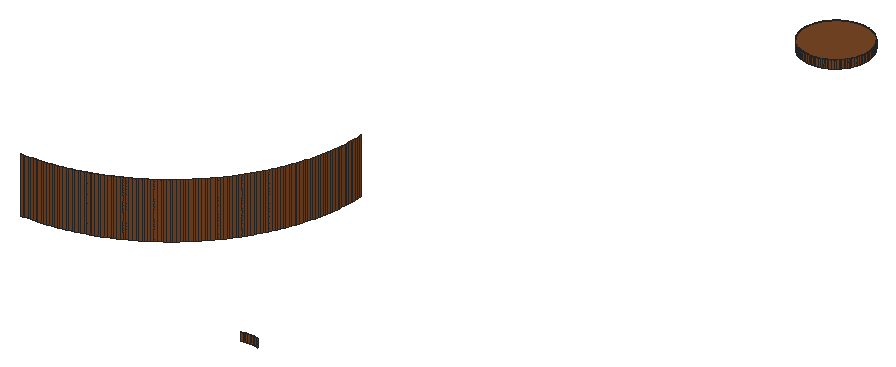
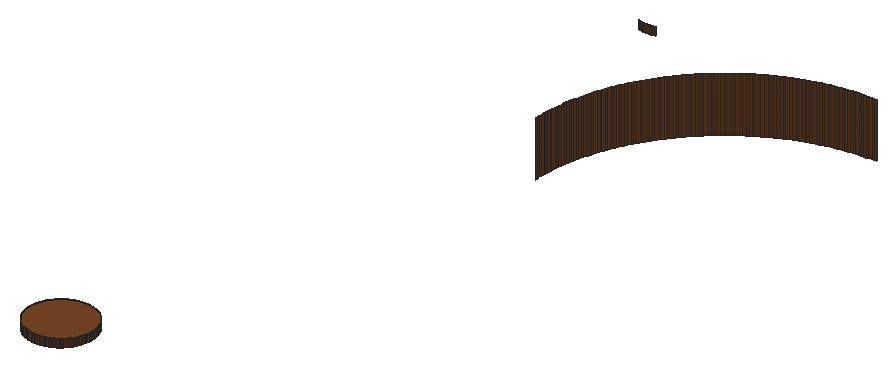
# SketchUp Ruby script. Lengths in inches.
U = 1.inch
M = Sketchup.active_model
def pt(a) = Geom::Point3d.new(a.map { |v| v * U })
def face(e, loops, mat)
  f = e.add_face(loops[0].map { |a| pt(a) })
  loops[1..].each { |l| e.add_face(l.map { |a| pt(a) }).erase! }
  f.material = f.back_material = mat if mat
  f
end
# faces: each face lists its corners as indices into pts; further lists are holes
def faces(e, pts, list, mat = nil) = list.each { |f| face(e, (f[0].is_a?(Array) ? f : [f]).map { |l| l.map { |i| pts[i] } }, mat) }
# xy, xz, yz: faces in a plane at the given z, y or x. An outline is a flat list of corners, or four numbers for a rectangle; further outlines are holes
def ring(l) = l.size == 4 ? [[l[0], l[1]], [l[2], l[1]], [l[2], l[3]], [l[0], l[3]]] : l.each_slice(2).to_a
def flat(e, list, mat, &to3) = list.each { |f| face(e, (f[0].is_a?(Array) ? f : [f]).map { |l| ring(l).map { |u, v| to3.(u, v) } }, mat) }
def xy(e, z, list, mat = nil) = flat(e, list, mat) { |x, y| [x, y, z] }
def xz(e, y, list, mat = nil) = flat(e, list, mat) { |x, z| [x, y, z] }
def yz(e, x, list, mat = nil) = flat(e, list, mat) { |y, z| [x, y, z] }
def lines(e, pts, list) = list.each { |a, b| e.add_line(pt(pts[a]), pt(pts[b])) }
# prism: a flat outline (further loops are holes) pulled along v
def prism(e, loops, v, mat = nil)
  f = face(e, loops, mat); d = Geom::Vector3d.new(v.map { |x| x * U })
  f.pushpull(f.normal.samedirection?(d) ? d.length : -d.length)
end
def box(e, o, s, mat = nil) = prism(e, [[o, [o[0] + s[0], o[1], o[2]], [o[0] + s[0], o[1] + s[1], o[2]], [o[0], o[1] + s[1], o[2]]]], [0, 0, s[2]], mat)
def at(x, y, z, deg = 0) = Geom::Transformation.translation(pt([x, y, z])) * Geom::Transformation.rotation(ORIGIN, Z_AXIS, deg.degrees)
def axes(o, x, y, z) = Geom::Transformation.new([*x, 0, *y, 0, *z, 0, *pt(o).to_a, 1])
def part(name) = M.definitions.add(name)
# library, detail: a bought-in or finely detailed component or shape, given as its bounding box
def library(name, o, s) = part(name).tap { |d| box(d.entities, o, s) }
def detail(e, o, s) = box(e.add_group.entities, o, s)
def put(e, d, t, mat = nil) = e.add_instance(d, t).tap { |i| i.material = mat if mat }
def group(e, t, mat = nil) = e.add_group.tap { |g| g.transformation = t; g.material = mat if mat }.entities
root = M.entities
M.materials.add("[Wood Veneer 01]3").color = [120, 70, 37]
xy(root,118.5,[[146.99,81.33,146.9,81.34,146.82,81.34,146.74,81.35,146.65,81.36,146.41,81.42,146.17,81.51,146.1,81.55,146.02,81.59,145.95,81.63,145.88,81.68,145.8125,81.72,145.75,81.77,145.68,81.83,145.62,81.89,145.5625,81.94,145.5,82.01,145.45,82.07,145.4,82.14,145.35,82.2,145.3,82.27,145.26,82.35,145.18,82.49,145.09,82.73,145.03,82.97,145.02,83.06,145,83.22,145,83.47,145.01,83.56,145.02,83.64,145.1,83.96,145.16,84.12,145.2,84.2,145.23,84.27,145.27,84.35,145.37,84.49,145.42,84.55,145.47,84.62,145.52,84.68,145.7,84.86,145.84,84.96,145.9,85.01,145.98,85.05,146.05,85.09,146.2,85.17,146.36,85.23,146.68,85.31,146.76,85.32,146.85,85.33,147.18,85.33,147.26,85.32,147.35,85.3,147.43,85.29,147.51,85.27,147.59,85.24,147.67,85.22,147.75,85.1875,147.83,85.15,147.9,85.12,147.98,85.08,148.05,85.04,148.12,84.99,148.1875,84.94,148.25,84.89,148.32,84.84,148.38,84.78,148.4375,84.72,148.5,84.66,148.55,84.6,148.7,84.39,148.78,84.25,148.82,84.17,148.85,84.1,148.88,84.02,148.91,83.9375,148.93,83.86,148.95,83.78,148.97,83.69,148.99,83.53,149,83.44,149,83.19,148.98,83.03,148.96,82.94,148.9,82.7,148.84,82.55,148.8,82.47,148.77,82.39,148.73,82.32,148.58,82.11,148.53,82.05,148.48,81.98,148.42,81.92,148.36,81.87,148.3,81.81,148.16,81.71,148.1,81.66,148.02,81.62,147.95,81.57,147.875,81.54,147.8,81.5,147.56,81.41,147.48,81.39,147.32,81.36,147.24,81.35,147.15,81.34,147.07,81.33]],"[Wood Veneer 01]3")
xz(root,41.99,[[142.76,118,142.85,118.5]],"[Wood Veneer 01]3")
xz(root,42,[[142.93,118,143.01,118.5],[143.01,118,143.1,118.5]],"[Wood Veneer 01]3")
xz(root,45,[[126,118,126.16,121.5],[126.16,118,126.3125,121.5]],"[Wood Veneer 01]3")
xz(root,81.33,[[146.99,118,147.07,118.5]],"[Wood Veneer 01]3")
xz(root,81.34,[[146.82,118,146.9,118.5]],"[Wood Veneer 01]3")
xz(root,85.33,[[146.85,118,146.93,118.5],[146.93,118,147.01,118.5],[147.01,118,147.1,118.5],[147.1,118,147.18,118.5]],"[Wood Veneer 01]3")
yz(root,138,[[56.6875,118,56.84,121.5],[56.84,118,57,121.5]],"[Wood Veneer 01]3")
yz(root,145,[[83.22,118,83.31,118.5],[83.31,118,83.39,118.5],[83.39,118,83.47,118.5]],"[Wood Veneer 01]3")
yz(root,149,[[83.19,118,83.28,118.5],[83.28,118,83.36,118.5],[83.36,118,83.44,118.5]],"[Wood Veneer 01]3")
p = [[142.44,41.92,118],[142.52,41.94,118],[142.52,41.94,118.5],[142.44,41.92,118.5],[142.6,41.96,118],[142.6,41.96,118.5],
  [143.43,41.95,118],[143.51,41.93,118],[143.51,41.93,118.5],[143.43,41.95,118.5],[142.68,41.97,118],[142.68,41.97,118.5],
  [142.76,41.99,118],[142.76,41.99,118.5],[142.85,41.99,118],[142.93,42,118],[142.93,42,118.5],[142.85,41.99,118.5],
  [143.1,42,118],[143.18,41.99,118],[143.18,41.99,118.5],[143.1,42,118.5],[143.26,41.98,118],[143.26,41.98,118.5],
  [143.35,41.97,118],[143.35,41.97,118.5],[126.3125,45,118],[126.3125,45,121],[126.3125,45,121.5],[126.47,45.01,121.5],
  [126.47,45.01,121],[126.47,45.01,118],[126.63,45.02,121.5],[126.63,45.02,121],[126.63,45.02,118],[126.78,45.03,121.5],
  [126.78,45.03,121],[126.78,45.03,118],[126.94,45.04,121.5],[126.94,45.04,121],[126.94,45.04,118],[127.1,45.05,121.5],
  [127.1,45.05,121],[127.1,45.05,118],[127.25,45.07,121.5],[127.25,45.07,121],[127.25,45.07,118],[127.41,45.08,121.5],
  [127.41,45.08,121],[127.41,45.08,118],[127.57,45.1,121.5],[127.57,45.1,121],[127.57,45.1,118],[127.72,45.125,121.5],
  [127.72,45.125,121],[127.72,45.125,118],[127.88,45.15,121.5],[127.88,45.15,121],[127.88,45.15,118],[128.03,45.17,121.5],
  [128.03,45.17,121],[128.03,45.17,118],[128.1875,45.2,121.5],[128.1875,45.2,121],[128.1875,45.2,118],[128.34,45.23,121.5],
  [128.34,45.23,121],[128.34,45.23,118],[128.49,45.26,121.5],[128.49,45.26,121],[128.49,45.26,118],[128.65,45.3,121.5],
  [128.65,45.3,121],[128.65,45.3,118],[128.8,45.33,121.5],[128.8,45.33,121],[128.8,45.33,118],[128.95,45.37,121.5],
  [128.95,45.37,121],[128.95,45.37,118],[129.11,45.41,121.5],[129.11,45.41,121],[129.11,45.41,118],[129.26,45.45,121.5],
  [129.26,45.45,121],[129.26,45.45,118],[129.41,45.49,121.5],[129.41,45.49,121],[129.41,45.49,118],[129.56,45.54,121.5],
  [129.56,45.54,121],[129.56,45.54,118],[129.71,45.59,121.5],[129.71,45.59,121],[129.71,45.59,118],[129.86,45.64,121.5],
  [129.86,45.64,121],[129.86,45.64,118],[130.01,45.6875,121.5],[130.01,45.6875,121],[130.01,45.6875,118],[130.15,45.74,121.5],
  [130.15,45.74,121],[130.15,45.74,118],[130.3,45.8,121.5],[130.3,45.8,121],[130.3,45.8,118],[130.45,45.85,121.5],
  [130.45,45.85,121],[130.45,45.85,118],[130.59,45.91,121.5],[130.59,45.91,121],[130.59,45.91,118],[130.74,45.97,121.5],
  [130.74,45.97,121],[130.74,45.97,118],[130.88,46.04,121.5],[130.88,46.04,121],[130.88,46.04,118],[131.02,46.1,121.5],
  [131.02,46.1,121],[131.02,46.1,118],[131.17,46.17,121.5],[131.17,46.17,121],[131.17,46.17,118],[131.31,46.24,121.5],
  [131.31,46.24,121],[131.31,46.24,118],[131.45,46.31,121.5],[131.45,46.31,121],[131.45,46.31,118],[131.59,46.38,121.5],
  [131.59,46.38,121],[131.59,46.38,118],[131.73,46.45,121.5],[131.73,46.45,121],[131.73,46.45,118],[131.86,46.53,121.5],
  [131.86,46.53,121],[131.86,46.53,118],[132,46.61,121.5],[132,46.61,121],[132,46.61,118],[132.14,46.6875,121.5],
  [132.14,46.6875,121],[132.14,46.6875,118],[132.27,46.77,121.5],[132.27,46.77,121],[132.27,46.77,118],[132.4,46.85,121.5],
  [132.4,46.85,121],[132.4,46.85,118],[132.54,46.9375,121.5],[132.54,46.9375,121],[132.54,46.9375,118],[132.67,47.02,121.5],
  [132.67,47.02,121],[132.67,47.02,118],[132.8,47.11,121.5],[132.8,47.11,121],[132.8,47.11,118],[132.93,47.2,121.5],
  [132.93,47.2,121],[132.93,47.2,118],[133.05,47.29,121.5],[133.05,47.29,121],[133.05,47.29,118],[133.18,47.38,121.5],
  [133.18,47.38,121],[133.18,47.38,118],[133.31,47.48,121.5],[133.31,47.48,121],[133.31,47.48,118],[133.43,47.58,121.5],
  [133.43,47.58,121],[133.43,47.58,118],[133.55,47.67,121.5],[133.55,47.67,121],[133.55,47.67,118],[133.67,47.77,121.5],
  [133.67,47.77,121],[133.67,47.77,118],[133.79,47.875,121.5],[133.79,47.875,121],[133.79,47.875,118],[133.91,47.98,121.5],
  [133.91,47.98,121],[133.91,47.98,118],[134.03,48.08,121.5],[134.03,48.08,121],[134.03,48.08,118],[134.15,48.1875,121.5],
  [134.15,48.1875,121],[134.15,48.1875,118],[134.26,48.3,121.5],[134.26,48.3,121],[134.26,48.3,118],[134.375,48.4,121.5],
  [134.375,48.4,121],[134.375,48.4,118],[134.49,48.51,121.5],[134.49,48.51,121],[134.49,48.51,118],[134.6,48.625,121.5],
  [134.6,48.625,121],[134.6,48.625,118],[134.7,48.74,121.5],[134.7,48.74,121],[134.7,48.74,118],[134.8125,48.85,121.5],
  [134.8125,48.85,121],[134.8125,48.85,118],[134.92,48.97,121.5],[134.92,48.97,121],[134.92,48.97,118],[135.02,49.09,121.5],
  [135.02,49.09,121],[135.02,49.09,118],[135.125,49.21,121.5],[135.125,49.21,121],[135.125,49.21,118],[135.23,49.33,121.5],
  [135.23,49.33,121],[135.23,49.33,118],[135.33,49.45,121.5],[135.33,49.45,121],[135.33,49.45,118],[135.42,49.57,121.5],
  [135.42,49.57,121],[135.42,49.57,118],[135.52,49.69,121.5],[135.52,49.69,121],[135.52,49.69,118],[135.62,49.82,121.5],
  [135.62,49.82,121],[135.62,49.82,118],[135.71,49.95,121.5],[135.71,49.95,121],[135.71,49.95,118],[135.8,50.07,121.5],
  [135.8,50.07,121],[135.8,50.07,118],[135.89,50.2,121.5],[135.89,50.2,121],[135.89,50.2,118],[135.98,50.33,121.5],
  [135.98,50.33,121],[135.98,50.33,118],[136.0625,50.46,121.5],[136.0625,50.46,121],[136.0625,50.46,118],[136.15,50.6,121.5],
  [136.15,50.6,121],[136.15,50.6,118],[136.23,50.73,121.5],[136.23,50.73,121],[136.23,50.73,118],[136.3125,50.86,121.5],
  [136.3125,50.86,121],[136.3125,50.86,118],[136.39,51,121.5],[136.39,51,121],[136.39,51,118],[136.47,51.14,121.5],
  [136.47,51.14,121],[136.47,51.14,118],[136.55,51.27,121.5],[136.55,51.27,121],[136.55,51.27,118],[136.62,51.41,121.5],
  [136.62,51.41,121],[136.62,51.41,118],[136.69,51.55,121.5],[136.69,51.55,121],[136.69,51.55,118],[136.76,51.69,121.5],
  [136.76,51.69,121],[136.76,51.69,118],[136.83,51.83,121.5],[136.83,51.83,121],[136.83,51.83,118],[136.9,51.98,121.5],
  [136.9,51.98,121],[136.9,51.98,118],[136.96,52.12,121.5],[136.96,52.12,121],[136.96,52.12,118],[137.03,52.26,121.5],
  [137.03,52.26,121],[137.03,52.26,118],[137.09,52.41,121.5],[137.09,52.41,121],[137.09,52.41,118],[137.15,52.55,121.5],
  [137.15,52.55,121],[137.15,52.55,118],[137.2,52.7,121.5],[137.2,52.7,121],[137.2,52.7,118],[137.26,52.85,121.5],
  [137.26,52.85,121],[137.26,52.85,118],[137.3125,52.99,121.5],[137.3125,52.99,121],[137.3125,52.99,118],[137.36,53.14,121.5],
  [137.36,53.14,121],[137.36,53.14,118],[137.41,53.29,121.5],[137.41,53.29,121],[137.41,53.29,118],[137.46,53.44,121.5],
  [137.46,53.44,121],[137.46,53.44,118],[137.51,53.59,121.5],[137.51,53.59,121],[137.51,53.59,118],[137.55,53.74,121.5],
  [137.55,53.74,121],[137.55,53.74,118],[137.59,53.89,121.5],[137.59,53.89,121],[137.59,53.89,118],[137.63,54.05,121.5],
  [137.63,54.05,121],[137.63,54.05,118],[137.67,54.2,121.5],[137.67,54.2,121],[137.67,54.2,118],[137.7,54.35,121.5],
  [137.7,54.35,121],[137.7,54.35,118],[137.74,54.51,121.5],[137.74,54.51,121],[137.74,54.51,118],[137.77,54.66,121.5],
  [137.77,54.66,121],[137.77,54.66,118],[137.8,54.8125,121.5],[137.8,54.8125,121],[137.8,54.8125,118],[137.83,54.97,121.5],
  [137.83,54.97,121],[137.83,54.97,118],[137.85,55.12,121.5],[137.85,55.12,121],[137.85,55.12,118],[137.875,55.28,121.5],
  [137.875,55.28,121],[137.875,55.28,118],[137.9,55.43,121.5],[137.9,55.43,121],[137.9,55.43,118],[137.92,55.59,121.5],
  [137.92,55.59,121],[137.92,55.59,118],[137.93,55.75,121.5],[137.93,55.75,121],[137.93,55.75,118],[137.95,55.9,121.5],
  [137.95,55.9,121],[137.95,55.9,118],[137.96,56.06,121.5],[137.96,56.06,121],[137.96,56.06,118],[137.97,56.22,121.5],
  [137.97,56.22,121],[137.97,56.22,118],[137.98,56.37,121.5],[137.98,56.37,121],[137.98,56.37,118],[137.99,56.53,121.5],
  [137.99,56.53,121],[137.99,56.53,118],[138,56.6875,121.5],[138,56.6875,121],[138,56.6875,118],[146.82,81.34,118],
  [146.74,81.35,118],[146.74,81.35,118.5],[146.82,81.34,118.5],[146.99,81.33,118],[146.9,81.34,118],[146.9,81.34,118.5],
  [146.99,81.33,118.5],[147.15,81.34,118],[147.07,81.33,118],[147.07,81.33,118.5],[147.15,81.34,118.5],[147.24,81.35,118],
  [147.24,81.35,118.5],[147.32,81.36,118],[147.32,81.36,118.5],[146.41,81.42,118],[146.33,81.45,118],[146.33,81.45,118.5],
  [146.41,81.42,118.5],[146.25,81.48,118],[146.25,81.48,118.5],[146.49,81.4,118],[146.49,81.4,118.5],[146.57,81.38,118],
  [146.57,81.38,118.5],[146.65,81.36,118],[146.65,81.36,118.5],[147.4,81.375,118],[147.4,81.375,118.5],[147.48,81.39,118],
  [147.48,81.39,118.5],[147.56,81.41,118],[147.56,81.41,118.5],[147.64,81.44,118],[147.64,81.44,118.5],[147.72,81.47,118],
  [147.72,81.47,118.5],[146.1,81.55,118],[146.02,81.59,118],[146.02,81.59,118.5],[146.1,81.55,118.5],[146.17,81.51,118],
  [146.17,81.51,118.5],[147.8,81.5,118],[147.8,81.5,118.5],[147.875,81.54,118],[147.875,81.54,118.5],[147.95,81.57,118],
  [147.95,81.57,118.5],[145.95,81.63,118],[145.88,81.68,118],[145.88,81.68,118.5],[145.95,81.63,118.5],[148.02,81.62,118],
  [148.02,81.62,118.5],[148.1,81.66,118],[148.1,81.66,118.5],[145.8125,81.72,118],[145.75,81.77,118],[145.75,81.77,118.5],
  [145.8125,81.72,118.5],[148.16,81.71,118],[148.16,81.71,118.5],[148.23,81.76,118],[148.23,81.76,118.5],[145.68,81.83,118],
  [145.62,81.89,118],[145.62,81.89,118.5],[145.68,81.83,118.5],[148.3,81.81,118],[148.3,81.81,118.5],[148.36,81.87,118],
  [148.36,81.87,118.5],[145.5625,81.94,118],[145.5,82.01,118],[145.5,82.01,118.5],[145.5625,81.94,118.5],[148.42,81.92,118],
  [148.42,81.92,118.5],[148.48,81.98,118],[148.48,81.98,118.5],[145.45,82.07,118],[145.45,82.07,118.5],[148.53,82.05,118],
  [148.53,82.05,118.5],[148.58,82.11,118],[148.58,82.11,118.5],[145.4,82.14,118],[145.35,82.2,118],[145.35,82.2,118.5],
  [145.4,82.14,118.5],[148.63,82.18,118],[148.63,82.18,118.5],[145.3,82.27,118],[145.3,82.27,118.5],[148.68,82.25,118],
  [148.68,82.25,118.5],[148.73,82.32,118],[148.73,82.32,118.5],[145.26,82.35,118],[145.22,82.42,118],[145.22,82.42,118.5],
  [145.26,82.35,118.5],[148.77,82.39,118],[148.77,82.39,118.5],[145.18,82.49,118],[145.18,82.49,118.5],[148.8,82.47,118],
  [148.8,82.47,118.5],[145.15,82.57,118],[145.15,82.57,118.5],[148.84,82.55,118],[148.84,82.55,118.5],[148.87,82.625,118],
  [148.87,82.625,118.5],[145.12,82.65,118],[145.12,82.65,118.5],[145.09,82.73,118],[145.09,82.73,118.5],[148.9,82.7,118],
  [148.9,82.7,118.5],[145.07,82.81,118],[145.07,82.81,118.5],[148.92,82.78,118],[148.92,82.78,118.5],[145.05,82.89,118],
  [145.05,82.89,118.5],[148.94,82.86,118],[148.94,82.86,118.5],[145.03,82.97,118],[145.03,82.97,118.5],[148.96,82.94,118],
  [148.96,82.94,118.5],[148.98,83.03,118],[148.98,83.03,118.5],[145.02,83.06,118],[145.02,83.06,118.5],[148.99,83.11,118],
  [148.99,83.11,118.5],[145.01,83.14,118],[145.01,83.14,118.5],[145,83.22,118],[145,83.22,118.5],[149,83.19,118],
  [149,83.19,118.5],[148.99,83.53,118],[149,83.44,118],[149,83.44,118.5],[148.99,83.53,118.5],[145,83.47,118],
  [145.01,83.56,118],[145.01,83.56,118.5],[145,83.47,118.5],[148.98,83.61,118],[148.98,83.61,118.5],[145.02,83.64,118],
  [145.02,83.64,118.5],[145.04,83.72,118],[145.04,83.72,118.5],[148.97,83.69,118],[148.97,83.69,118.5],[145.06,83.8,118],
  [145.06,83.8,118.5],[148.95,83.78,118],[148.95,83.78,118.5],[145.08,83.88,118],[145.08,83.88,118.5],[148.93,83.86,118],
  [148.93,83.86,118.5],[145.1,83.96,118],[145.1,83.96,118.5],[148.91,83.9375,118],[148.91,83.9375,118.5],[148.88,84.02,118],
  [148.88,84.02,118.5],[145.13,84.04,118],[145.13,84.04,118.5],[145.16,84.12,118],[145.16,84.12,118.5],[148.85,84.1,118],
  [148.85,84.1,118.5],[145.2,84.2,118],[145.2,84.2,118.5],[148.82,84.17,118],[148.82,84.17,118.5],[145.23,84.27,118],
  [145.23,84.27,118.5],[148.74,84.32,118],[148.78,84.25,118],[148.78,84.25,118.5],[148.74,84.32,118.5],[145.27,84.35,118],
  [145.27,84.35,118.5],[145.32,84.42,118],[145.32,84.42,118.5],[148.7,84.39,118],[148.7,84.39,118.5],[145.37,84.49,118],
  [145.37,84.49,118.5],[148.65,84.46,118],[148.65,84.46,118.5],[145.42,84.55,118],[145.42,84.55,118.5],[148.55,84.6,118],
  [148.6,84.53,118],[148.6,84.53,118.5],[148.55,84.6,118.5],[145.47,84.62,118],[145.47,84.62,118.5],[145.52,84.68,118],
  [145.52,84.68,118.5],[148.5,84.66,118],[148.5,84.66,118.5],[145.58,84.74,118],[145.58,84.74,118.5],[145.64,84.8,118],
  [145.64,84.8,118.5],[148.4375,84.72,118],[148.4375,84.72,118.5],[148.38,84.78,118],[148.38,84.78,118.5],[145.7,84.86,118],
  [145.7,84.86,118.5],[148.32,84.84,118],[148.32,84.84,118.5],[148.25,84.89,118],[148.25,84.89,118.5],[145.77,84.91,118],
  [145.77,84.91,118.5],[145.84,84.96,118],[145.84,84.96,118.5],[148.12,84.99,118],[148.1875,84.94,118],[148.1875,84.94,118.5],
  [148.12,84.99,118.5],[145.9,85.01,118],[145.9,85.01,118.5],[145.98,85.05,118],[145.98,85.05,118.5],[148.05,85.04,118],
  [148.05,85.04,118.5],[147.98,85.08,118],[147.98,85.08,118.5],[146.05,85.09,118],[146.05,85.09,118.5],[146.125,85.13,118],
  [146.125,85.13,118.5],[146.2,85.17,118],[146.2,85.17,118.5],[147.83,85.15,118],[147.9,85.12,118],[147.9,85.12,118.5],
  [147.83,85.15,118.5],[146.28,85.2,118],[146.28,85.2,118.5],[146.36,85.23,118],[146.36,85.23,118.5],[146.44,85.25,118],
  [146.44,85.25,118.5],[147.51,85.27,118],[147.59,85.24,118],[147.59,85.24,118.5],[147.51,85.27,118.5],[147.67,85.22,118],
  [147.67,85.22,118.5],[147.75,85.1875,118],[147.75,85.1875,118.5],[146.52,85.27,118],[146.52,85.27,118.5],[146.6,85.29,118],
  [146.6,85.29,118.5],[146.68,85.31,118],[146.68,85.31,118.5],[146.76,85.32,118],[146.76,85.32,118.5],[146.85,85.33,118],
  [146.85,85.33,118.5],[147.18,85.33,118],[147.26,85.32,118],[147.26,85.32,118.5],[147.18,85.33,118.5],[147.35,85.3,118],
  [147.43,85.29,118],[147.43,85.29,118.5],[147.35,85.3,118.5]]
faces(root,p,[[0,1,2,3],[1,4,5,2],[6,7,8,9],[4,10,11,5],[10,12,13,11],[14,15,16,17],[18,19,20,21],[19,22,23,20],
  [24,6,9,25],[22,24,25,23],[26,27,28,29,30,31],[31,30,29,32,33,34],[34,33,32,35,36,37],[37,36,35,38,39,40],[40,39,38,41,42,43],[43,42,41,44,45,46],
  [46,45,44,47,48,49],[49,48,47,50,51,52],[52,51,50,53,54,55],[55,54,53,56,57,58],[58,57,56,59,60,61],[61,60,59,62,63,64],[64,63,62,65,66,67],[67,66,65,68,69,70],
  [70,69,68,71,72,73],[73,72,71,74,75,76],[76,75,74,77,78,79],[79,78,77,80,81,82],[82,81,80,83,84,85],[85,84,83,86,87,88],[88,87,86,89,90,91],[91,90,89,92,93,94],
  [94,93,92,95,96,97],[97,96,95,98,99,100],[100,99,98,101,102,103],[103,102,101,104,105,106],[106,105,104,107,108,109],[109,108,107,110,111,112],[112,111,110,113,114,115],[115,114,113,116,117,118],
  [118,117,116,119,120,121],[121,120,119,122,123,124],[124,123,122,125,126,127],[127,126,125,128,129,130],[130,129,128,131,132,133],[133,132,131,134,135,136],[136,135,134,137,138,139],[139,138,137,140,141,142],
  [142,141,140,143,144,145],[145,144,143,146,147,148],[148,147,146,149,150,151],[151,150,149,152,153,154],[154,153,152,155,156,157],[157,156,155,158,159,160],[160,159,158,161,162,163],[163,162,161,164,165,166],
  [166,165,164,167,168,169],[169,168,167,170,171,172],[172,171,170,173,174,175],[175,174,173,176,177,178],[178,177,176,179,180,181],[181,180,179,182,183,184],[184,183,182,185,186,187],[187,186,185,188,189,190],
  [190,189,188,191,192,193],[193,192,191,194,195,196],[196,195,194,197,198,199],[199,198,197,200,201,202],[202,201,200,203,204,205],[205,204,203,206,207,208],[208,207,206,209,210,211],[211,210,209,212,213,214],
  [214,213,212,215,216,217],[217,216,215,218,219,220],[220,219,218,221,222,223],[223,222,221,224,225,226],[226,225,224,227,228,229],[229,228,227,230,231,232],[232,231,230,233,234,235],[235,234,233,236,237,238],
  [238,237,236,239,240,241],[241,240,239,242,243,244],[244,243,242,245,246,247],[247,246,245,248,249,250],[250,249,248,251,252,253],[253,252,251,254,255,256],[256,255,254,257,258,259],[259,258,257,260,261,262],
  [262,261,260,263,264,265],[265,264,263,266,267,268],[268,267,266,269,270,271],[271,270,269,272,273,274],[274,273,272,275,276,277],[277,276,275,278,279,280],[280,279,278,281,282,283],[283,282,281,284,285,286],
  [286,285,284,287,288,289],[289,288,287,290,291,292],[292,291,290,293,294,295],[295,294,293,296,297,298],[298,297,296,299,300,301],[301,300,299,302,303,304],[304,303,302,305,306,307],[307,306,305,308,309,310],
  [310,309,308,311,312,313],[313,312,311,314,315,316],[316,315,314,317,318,319],[319,318,317,320,321,322],[322,321,320,323,324,325],[325,324,323,326,327,328],[328,327,326,329,330,331],[331,330,329,332,333,334],
  [334,333,332,335,336,337],[337,336,335,338,339,340],[340,339,338,341,342,343],[343,342,341,344,345,346],[346,345,344,347,348,349],[349,348,347,350,351,352],[352,351,350,353,354,355],[355,354,353,356,357,358],
  [358,357,356,359,360,361],[361,360,359,362,363,364],[364,363,362,365,366,367],[367,366,365,368,369,370],[370,369,368,371,372,373],[373,372,371,374,375,376],[377,378,379,380],[381,382,383,384],
  [385,386,387,388],[389,385,388,390],[391,389,390,392],[393,394,395,396],[394,397,398,395],[399,393,396,400],[401,399,400,402],[403,401,402,404],
  [378,403,404,379],[405,391,392,406],[407,405,406,408],[409,407,408,410],[411,409,410,412],[413,411,412,414],[415,416,417,418],[419,415,418,420],
  [397,419,420,398],[421,413,414,422],[423,421,422,424],[425,423,424,426],[427,428,429,430],[416,427,430,417],[431,425,426,432],[433,431,432,434],
  [435,436,437,438],[428,435,438,429],[439,433,434,440],[441,439,440,442],[443,444,445,446],[436,443,446,437],[447,441,442,448],[449,447,448,450],
  [451,452,453,454],[444,451,454,445],[455,449,450,456],[457,455,456,458],[452,459,460,453],[461,457,458,462],[463,461,462,464],[465,466,467,468],
  [459,465,468,460],[469,463,464,470],[466,471,472,467],[473,469,470,474],[475,473,474,476],[477,478,479,480],[471,477,480,472],[481,475,476,482],
  [478,483,484,479],[485,481,482,486],[483,487,488,484],[489,485,486,490],[491,489,490,492],[487,493,494,488],[493,495,496,494],[497,491,492,498],
  [495,499,500,496],[501,497,498,502],[499,503,504,500],[505,501,502,506],[503,507,508,504],[509,505,506,510],[511,509,510,512],[507,513,514,508],
  [515,511,512,516],[513,517,518,514],[517,519,520,518],[521,515,516,522],[523,524,525,526],[527,528,529,530],[531,523,526,532],[528,533,534,529],
  [533,535,536,534],[537,531,532,538],[535,539,540,536],[541,537,538,542],[539,543,544,540],[545,541,542,546],[543,547,548,544],[549,545,546,550],
  [551,549,550,552],[547,553,554,548],[553,555,556,554],[557,551,552,558],[555,559,560,556],[561,557,558,562],[559,563,564,560],[565,566,567,568],
  [566,561,562,567],[563,569,570,564],[569,571,572,570],[573,565,568,574],[571,575,576,572],[577,573,574,578],[575,579,580,576],[581,582,583,584],
  [582,577,578,583],[579,585,586,580],[585,587,588,586],[589,581,584,590],[587,591,592,588],[591,593,594,592],[595,589,590,596],[597,595,596,598],
  [593,599,600,594],[601,597,598,602],[603,601,602,604],[599,605,606,600],[605,607,608,606],[609,610,611,612],[610,603,604,611],[607,613,614,608],
  [613,615,616,614],[617,609,612,618],[619,617,618,620],[615,621,622,616],[621,623,624,622],[623,625,626,624],[627,628,629,630],[628,619,620,629],
  [625,631,632,626],[631,633,634,632],[633,635,636,634],[637,638,639,640],[638,641,642,639],[643,627,630,644],[641,643,644,642],[635,645,646,636],
  [645,647,648,646],[647,649,650,648],[649,651,652,650],[651,653,654,652],[655,656,657,658],[659,660,661,662],[656,659,662,657],[660,637,640,661]],"[Wood Veneer 01]3")
